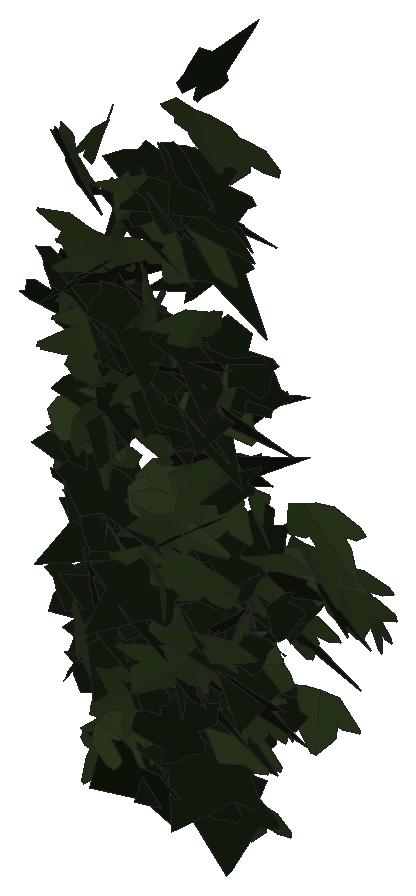
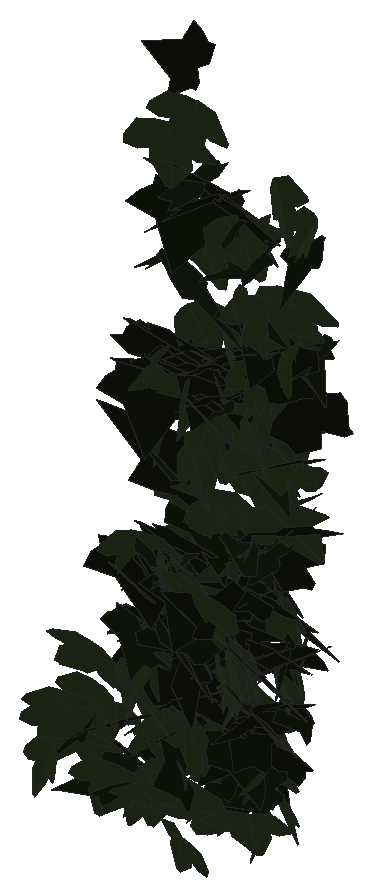
# SketchUp Ruby script. Lengths in millimetres.
U = 1.mm
M = Sketchup.active_model
def pt(a) = Geom::Point3d.new(a.map { |v| v * U })
def face(e, loops, mat)
  f = e.add_face(loops[0].map { |a| pt(a) })
  loops[1..].each { |l| e.add_face(l.map { |a| pt(a) }).erase! }
  f.material = f.back_material = mat if mat
  f
end
# faces: each face lists its corners as indices into pts; further lists are holes
def faces(e, pts, list, mat = nil) = list.each { |f| face(e, (f[0].is_a?(Array) ? f : [f]).map { |l| l.map { |i| pts[i] } }, mat) }
# xy, xz, yz: faces in a plane at the given z, y or x. An outline is a flat list of corners, or four numbers for a rectangle; further outlines are holes
def ring(l) = l.size == 4 ? [[l[0], l[1]], [l[2], l[1]], [l[2], l[3]], [l[0], l[3]]] : l.each_slice(2).to_a
def flat(e, list, mat, &to3) = list.each { |f| face(e, (f[0].is_a?(Array) ? f : [f]).map { |l| ring(l).map { |u, v| to3.(u, v) } }, mat) }
def xy(e, z, list, mat = nil) = flat(e, list, mat) { |x, y| [x, y, z] }
def xz(e, y, list, mat = nil) = flat(e, list, mat) { |x, z| [x, y, z] }
def yz(e, x, list, mat = nil) = flat(e, list, mat) { |y, z| [x, y, z] }
def lines(e, pts, list) = list.each { |a, b| e.add_line(pt(pts[a]), pt(pts[b])) }
# prism: a flat outline (further loops are holes) pulled along v
def prism(e, loops, v, mat = nil)
  f = face(e, loops, mat); d = Geom::Vector3d.new(v.map { |x| x * U })
  f.pushpull(f.normal.samedirection?(d) ? d.length : -d.length)
end
def box(e, o, s, mat = nil) = prism(e, [[o, [o[0] + s[0], o[1], o[2]], [o[0] + s[0], o[1] + s[1], o[2]], [o[0], o[1] + s[1], o[2]]]], [0, 0, s[2]], mat)
def at(x, y, z, deg = 0) = Geom::Transformation.translation(pt([x, y, z])) * Geom::Transformation.rotation(ORIGIN, Z_AXIS, deg.degrees)
def axes(o, x, y, z) = Geom::Transformation.new([*x, 0, *y, 0, *z, 0, *pt(o).to_a, 1])
def part(name) = M.definitions.add(name)
# library, detail: a bought-in or finely detailed component or shape, given as its bounding box
def library(name, o, s) = part(name).tap { |d| box(d.entities, o, s) }
def detail(e, o, s) = box(e.add_group.entities, o, s)
def put(e, d, t, mat = nil) = e.add_instance(d, t).tap { |i| i.material = mat if mat }
def group(e, t, mat = nil) = e.add_group.tap { |g| g.transformation = t; g.material = mat if mat }.entities
root = M.entities
M.materials.add("efeu1").color = [18, 25, 13]
M.materials.add("efeu2").color = [43, 57, 29]
c1 = part("ivyleaf_9")
p = [[39.1,54.8,31.7],[34.5,51.8,30.2],[-5.3,25.2,17.3],[-17.9,28.3,20.9],[-21.6,21.7,17],[-20.2,4.3,5.3],
  [-22.9,-0.3,2.5],[-17.1,-4,-0.6],[-2,-2.1,-1.2],[-0.7,-15.4,-10.1],[16.6,-22.3,-16.7],[21.1,-15.1,-12.5],
  [32.7,-10.7,-11],[46.1,-1.8,-6.6],[30.8,11.2,3.8]]
faces(c1.entities,p,[[0,1,2,3,4,5,6,7,8,9,10,11,12,13,14]],"efeu1")
c2 = part("ivyleaf_10")
p = [[0,12.8,-0.8],[-1.5,51.3,-10.9],[-4.9,51,-11.6],[-13.6,26.5,-7.3],[-13.2,15.9,-4.6],[-21.1,19.3,-7.2],
  [-29.5,16.3,-8.3],[-29.2,8.3,-6.2],[-19.7,-9.8,0.5],[-7.6,-13,4],[1,-12.2,5.8],[-0.4,51.1,-11.1],
  [-1.5,51.1,-10.9],[1,-12.4,5.9],[16.9,-12.4,3.5],[35.1,9.1,-5.1],[35,12.9,-6.1],[20.5,16.4,-4.9],
  [15.8,15,-3.8],[15.3,27.6,-7.1],[12.8,31.3,-7.8]]
faces(c2.entities,p,[[0,1,2,3,4,5,6,7,8,9,10],[11,12,0,13,14,15,16,17,18,19,20]],"efeu2")
put(root,c1,axes([3291.1,941.8,1866.9],[-1.63841,0.20506,-0.06305],[0.10638,-0.03734,-0.88465],[-0.3942,-0.86237,0.02331]))
put(root,c2,axes([3268.6,999.9,1657.1],[1.36446,0.42634,-0.10284],[-0.16436,-0.05598,-0.83411],[-0.81833,0.7221,-0.00394]))
put(root,c2,axes([3261,1111.8,1683.8],[1.21223,-0.44961,0.31681],[0.5749,-0.11914,-0.77639],[0.87479,0.70134,0.07122]))
put(root,c1,axes([3275.5,910.4,1743.9],[0.25103,0.30454,0.864],[0.47233,0.82839,-0.32988],[-1.67833,0.27868,0.03639]))
put(root,c2,axes([3294.5,926.8,1954.7],[-1.01266,-0.47157,0.54848],[-0.75507,-0.37907,-0.71079],[1.1511,-0.66351,0.01627]))
put(root,c2,axes([3274.6,938.9,1874.2],[0.99293,-0.73387,0.02376],[0.02687,-0.01911,-0.90042],[1.39718,0.52191,0.00043]))
put(root,c1,axes([3282.5,919,1826.6],[0.61878,-0.07581,-0.86332],[-1.36691,0.49246,-0.31372],[0.92307,0.78007,0.11416]))
put(root,c2,axes([3278.7,920.6,2128],[-0.11991,-0.82511,0.44369],[0.11724,-0.44737,-0.82322],[1.77912,-0.02613,0.08415]))
put(root,c2,axes([3273.8,968.6,1633.3],[-0.46378,0.81359,-0.01001],[-0.00783,-0.01168,-0.84927],[-1.54853,-0.24361,0.00729]))
put(root,c1,axes([3258,938.2,1814],[0.51924,-0.7897,-0.36067],[0.0588,0.38665,-0.82322],[1.65124,0.23456,0.14273]))
put(root,c1,axes([3245.1,924.3,2070.7],[1.86809,-0.02971,-0.34505],[0.65849,0.12956,0.97308],[0.02888,-1.03233,0.13205]))
put(root,c1,axes([3278.6,892.7,2249.9],[1.08597,-0.13273,-0.74714],[-1.20074,0.43646,-0.55937],[0.80251,0.83266,0.17411]))
put(root,c2,axes([3282,936.3,1650.5],[0.88369,-0.7013,-0.10271],[-0.10379,0.08708,-0.84108],[1.34496,0.4675,0.00258]))
put(root,c2,axes([3280.2,932.8,1781.1],[0.36461,-0.8497,0.28444],[0.16256,-0.27223,-0.87074],[1.69759,0.20857,0.02229]))
put(root,c2,axes([3280.7,935.3,1862.7],[-1.24826,0.57855,-0.19807],[0.06738,-0.25405,-0.85926],[-1.16188,-0.63629,0.16297]))
put(root,c2,axes([3289.5,919,2059.9],[-0.88419,-0.79522,0.11666],[-0.02452,-0.12737,-0.91947],[1.52947,-0.46176,0.0527]))
put(root,c2,axes([3279.4,959.6,1655.2],[-0.30491,0.82154,-0.12098],[0.02656,-0.12053,-0.83696],[-1.58019,-0.16055,0.00928]))
put(root,c1,axes([3269.8,945,1754.5],[0.52384,-0.21759,-0.79415],[-0.233,0.81722,-0.26634],[1.5497,0.19642,0.2284]))
put(root,c1,axes([3284.4,1083.7,1737.7],[0.29329,0.23543,0.82329],[0.48535,0.78594,-0.27248],[-1.55574,0.28958,0.0702]))
put(root,c1,axes([3285.8,933.1,1942.7],[-0.99855,-0.73699,0.09525],[-0.04457,-0.10014,-0.90384],[1.4136,-0.52376,0.03878]))
put(root,c1,axes([3301.4,885,2144.4],[-0.25789,0.93298,0.12548],[-0.0107,0.12597,-0.94269],[-1.79161,-0.13505,-0.01243]))
put(root,c2,axes([3281.1,968.4,1689.2],[-0.26334,0.83743,0.04284],[0.00062,0.04347,-0.84875],[-1.59589,-0.13817,-0.0074]))
put(root,c2,axes([3300.7,896.4,2178.8],[-1.69504,0.05393,0.30576],[-0.58094,0.01773,-0.89226],[-0.10803,-0.94148,0.00072]))
put(root,c1,axes([3263.5,970.7,1680.9],[1.19495,-0.56293,-0.03573],[0.04025,0.07691,-0.84025],[1.07278,0.62416,0.07132]))
put(root,c2,axes([3291,915.5,2065.8],[-1.09684,-0.75007,0.02522],[0.13556,-0.08632,-0.93961],[1.4219,-0.57037,0.10903]))
put(root,c1,axes([3265.3,909,2130.1],[0.61208,-0.89231,0.10139],[0.09667,-0.08945,-0.94834],[1.70644,0.32513,0.01736]))
put(root,c2,axes([3285.1,888.8,2265.1],[-0.9256,0.81522,0.00802],[0.01029,0.01257,-0.9492],[-1.55156,-0.48624,-0.01108]))
put(root,c1,axes([3287.3,957.2,1750.5],[-0.68087,-0.74381,0.21767],[-0.18868,-0.19385,-0.82535],[1.46287,-0.3712,-0.00515]))
put(root,c1,axes([3318,956.8,1807],[-0.96334,0.64874,0.28351],[-0.41672,0.18798,-0.82107],[-1.28137,-0.54886,0.05388]))
put(root,c1,axes([3276,922,1946.9],[0.70388,-0.75674,-0.35005],[-0.31631,0.30835,-0.84218],[1.555,0.40527,-0.01286]))
put(root,c2,axes([3273.2,913.3,1782.4],[0.19932,-0.36689,0.82699],[1.12123,-0.60416,-0.34264],[1.30678,0.57434,0.16785]))
put(root,c1,axes([3270.6,959.7,1721.2],[-0.41494,-0.23195,-0.79436],[1.39421,0.32799,-0.29684],[0.73256,-0.75562,0.115]))
put(root,c2,axes([3281.8,905.4,1999.4],[0.82313,0.71572,0.44173],[0.40911,0.38615,-0.83613],[-1.54755,0.48277,0.01391]))
put(root,c2,axes([3302.1,883.4,2001.3],[0.17706,0.56348,0.72436],[-0.56728,0.70716,-0.51182],[-1.65192,-0.18244,0.2534]))
put(root,c1,axes([3313.5,966,1710.4],[-0.17603,0.83843,-0.1339],[0.00078,-0.13465,-0.8434],[-1.61592,-0.0914,0.01418]))
put(root,c1,axes([3323.1,959.9,1768],[-1.11865,0.61618,0.06786],[-0.11089,0.03819,-0.85141],[-1.17458,-0.59044,0.01575]))
put(root,c2,axes([3306.1,915.7,2093.8],[-0.93168,-0.7833,0.20194],[0.02648,-0.24416,-0.91333],[1.53929,-0.4699,0.13794]))
put(root,c2,axes([3308,929.5,2015.3],[-1.50879,-0.45023,-0.02683],[0.03169,0.025,-0.91159],[0.8578,-0.79282,-0.01351]))
put(root,c1,axes([3312.4,948.2,1814.8],[-1.60594,-0.19726,-0.18221],[0.36375,-0.0191,-0.86443],[0.35901,-0.86305,0.06078]))
put(root,c2,axes([3312.7,920.1,2106],[-1.39002,-0.58311,0.05549],[-0.08609,-0.03227,-0.93458],[1.11146,-0.73175,-0.003]))
put(root,c2,axes([3309,909.9,2154.5],[-0.96161,-0.80101,-0.05026],[0.12091,0.01929,-0.94606],[1.5227,-0.50739,0.04338]))
put(root,c1,axes([3288.1,933.6,1881.1],[0.5229,-0.80355,-0.27842],[-0.04352,0.2855,-0.84656],[1.61793,0.26738,0.06721]))
put(root,c2,axes([3308.5,956.7,1805.5],[0.54209,-0.82276,-0.06216],[0.00712,0.06705,-0.8703],[1.57032,0.28372,0.02541]))
put(root,c1,axes([3301.8,929.3,2007.2],[-0.68627,-0.83056,0.17307],[0.01472,-0.19126,-0.90176],[1.61461,-0.35128,0.08178]))
put(root,c1,axes([3270.7,917.7,1904.5],[1.12013,-0.42318,0.60133],[0.99188,-0.30329,-0.72352],[0.98723,0.78486,0.04464]))
put(root,c1,axes([3285.9,937.9,1915.6],[0.86805,-0.77566,-0.00192],[0.03362,0.01262,-0.89956],[1.47586,0.45593,0.02162]))
put(root,c2,axes([3317.8,912.2,1725.1],[1.03158,-0.50406,-0.50402],[-0.49408,0.45011,-0.72932],[1.26347,0.58756,0.12631]))
put(root,c1,axes([3271.5,922.9,2119.9],[1.27182,-0.28484,0.59393],[1.03542,-0.23831,-0.72641],[0.70675,0.8617,-0.00457]))
put(root,c1,axes([3299.2,926.7,1810.4],[-0.88287,-0.57428,-0.502],[0.6088,0.38692,-0.73822],[1.31786,-0.56347,0.00472]))
put(root,c1,axes([3297.5,966,1728.6],[1.66358,-0.12322,-0.31616],[-0.59212,0.05772,-0.88264],[0.2578,0.92772,0.01292]))
put(root,c2,axes([3300.2,1106.5,1726.4],[0.63414,0.76213,0.286],[0.20342,0.2654,-0.83175],[-1.53584,0.34983,0.00792]))
put(root,c2,axes([3315.1,892.7,2294.3],[0.05351,-0.9489,-0.20865],[0.02754,0.20912,-0.9491],[1.84888,0.02435,0.02018]))
put(root,c2,axes([3331.9,919.7,1689.6],[0.9452,-0.30401,-0.70783],[-1.09882,0.41067,-0.58147],[0.97065,0.76094,0.03102]))
put(root,c2,axes([3310.7,964.3,1772.3],[-0.82074,0.74065,0.05517],[-0.03569,0.05292,-0.85699],[-1.41307,-0.43153,-0.0104]))
put(root,c1,axes([3332.8,906.9,1995.8],[0.00541,0.77291,0.49877],[-0.51778,0.47716,-0.73788],[-1.67237,-0.14523,0.23006]))
put(root,c1,axes([3332.7,932,1912.6],[-0.90542,0.73736,-0.16871],[0.03254,-0.18877,-0.87325],[-1.43924,-0.46814,0.08639]))
put(root,c2,axes([3318.3,912.3,2169.1],[-1.57743,-0.45028,-0.04002],[0.04335,0.04187,-0.94289],[0.85926,-0.82874,-0.0259]))
put(root,c1,axes([3309.5,956.4,1801.4],[-0.55279,-0.77516,0.27355],[-0.00975,-0.28842,-0.82272],[1.56443,-0.2757,0.09153]))
put(root,c2,axes([3298.3,1082,1736.7],[-0.65088,0.40064,-0.69592],[0.79107,-0.55886,-0.526],[-1.3076,-0.53752,0.02819]))
put(root,c2,axes([3321.9,922,2044.9],[-0.22531,-0.92552,-0.06851],[0.0021,0.06893,-0.93303],[1.76626,-0.11814,-0.00763]))
put(root,c1,axes([3315.2,917.8,2123.7],[-0.7669,-0.85604,0.03989],[-0.02356,-0.03825,-0.94612],[1.63081,-0.40311,0.00509]))
put(root,c2,axes([3322.6,956.4,1799.8],[0.20143,-0.86488,-0.05368],[0.00093,0.05414,-0.8713],[1.6492,0.1056,0.00705]))
put(root,c1,axes([3319.6,897.8,2149.4],[0.80267,0.82441,0.1255],[0.13236,0.10537,-0.92592],[-1.58156,0.42722,-0.0138]))
put(root,c2,axes([3308.3,902.2,1987.4],[1.05478,-0.62262,0.39865],[0.68387,-0.20857,-0.8253],[1.22968,0.65006,0.11703]))
put(root,c1,axes([3303.2,892.5,1946.4],[0.69392,-0.78084,-0.35188],[0.04665,0.39179,-0.84402],[1.62936,0.32133,0.17402]))
put(root,c2,axes([3321.1,1097.7,1717.5],[-0.06378,0.79231,-0.3833],[-0.03994,-0.38419,-0.79232],[-1.67465,-0.02102,0.03349]))
put(root,c1,axes([3321.8,937.3,1662.9],[1.47789,-0.04593,-0.47015],[-0.89144,0.04255,-0.77778],[0.11669,0.90677,0.01268]))
put(root,c2,axes([3330.6,963.1,1790.5],[0.2883,-0.84444,-0.06332],[-0.00089,0.06424,-0.85785],[1.61165,0.15109,0.01085]))
put(root,c1,axes([3341.5,948,1710.3],[-1.55135,-0.24427,-0.00506],[0.00894,0.00197,-0.85094],[0.46491,-0.81514,-0.00054]))
put(root,c2,axes([3327.3,964.6,1716.1],[-0.83099,-0.6273,-0.38671],[0.37417,0.33404,-0.76384],[1.35167,-0.47812,-0.0263]))
put(root,c1,axes([3319.8,898,2033.5],[1.01509,-0.38539,-0.68611],[-0.71566,0.60329,-0.63118],[1.31566,0.62551,0.18603]))
put(root,c2,axes([3329.6,1090.7,1832.1],[-0.5716,0.79558,0.16934],[-0.12887,0.15543,-0.85035],[-1.5427,-0.30776,0.00829]))
put(root,c2,axes([3326.1,937.8,1906.9],[0.03479,0.8674,-0.26461],[0.00982,-0.26476,-0.86753],[-1.72592,0.01598,-0.01027]))
put(root,c1,axes([3325.3,961,1673.4],[1.17675,-0.36653,-0.46491],[-0.72696,0.26662,-0.71819],[0.86084,0.72619,0.02903]))
put(root,c2,axes([3331.2,929.8,1674.3],[-0.03022,-0.12607,-0.94432],[0.43653,0.91617,-0.12617],[1.75985,-0.22942,0.01508]))
put(root,c2,axes([3324.7,896.5,1698],[0.22969,0.64943,0.6144],[0.23018,0.60241,-0.66052],[-1.68583,0.17073,-0.00647]))
put(root,c2,axes([3323.4,953.8,1810.7],[1.30474,-0.47728,0.27133],[0.53186,-0.07027,-0.82967],[0.89939,0.73393,0.09701]))
put(root,c2,axes([3328.4,925.1,1985.2],[-0.00025,-1.00563,-0.30699],[0.08299,-0.30673,1.00477],[-1.9994,-0.0126,0.04174]))
put(root,c1,axes([3357.7,889.6,1677.5],[0.75096,0.07969,-0.90298],[-1.69747,-0.14185,-0.40226],[-0.30828,0.97517,0.01528]))
put(root,c1,axes([3343.5,1090.4,1820.9],[-1.268,0.29278,-0.48853],[0.83344,-0.21737,-0.72749],[-0.69306,-0.79705,0.01895]))
put(root,c1,axes([3347.2,952.1,1826.4],[-1.436,-0.4577,-0.00553],[0.01024,0.00179,-0.88249],[0.87109,-0.75454,0.00126]))
put(root,c2,axes([3344.7,934.9,1746.7],[-1.29077,-0.57029,-0.05161],[0.06775,0.03786,-0.88609],[1.08769,-0.67912,-0.00605]))
put(root,c2,axes([3335.4,955.6,1770.7],[-0.81675,0.70692,-0.22816],[0.18408,-0.20808,-0.82663],[-1.40172,-0.43924,0.02439]))
put(root,c1,axes([3323.9,904.9,2094.8],[0.92761,-0.71309,-0.3513],[-0.28245,0.3232,-0.86196],[1.4863,0.50647,0.05544]))
put(root,c1,axes([3320.5,926.8,1872.5],[1.70449,-0.12999,-0.0139],[-0.02625,0.00174,-0.90498],[0.24742,0.8957,-0.00026]))
put(root,c2,axes([3313.7,1005.5,1653.6],[0.47184,-0.07685,0.80375],[1.40922,0.3569,-0.19427],[-0.61275,0.76164,0.17213]))
put(root,c2,axes([3349.5,1111.7,1727.8],[-1.60537,0.0756,-0.06583],[0.12402,-0.01043,-0.84688],[-0.14498,-0.84601,0.00456]))
put(root,c2,axes([3357.5,929.6,1865.7],[-0.83895,-0.72991,0.3487],[-0.14927,-0.35668,-0.84575],[1.53229,-0.43438,0.10853]))
put(root,c2,axes([3362.3,908.8,2242],[-0.91767,-0.75284,0.31794],[-0.33781,-0.26387,-0.89399],[1.51822,-0.51376,-0.00674]))
put(root,c1,axes([3363.2,899.5,1854.1],[-1.61506,0.08778,-0.20637],[0.37512,-0.09341,-0.8502],[-0.20362,-0.86832,0.0706]))
put(root,c2,axes([3353.8,922,2031.2],[-0.87034,-0.8071,0.09596],[0.13713,-0.14992,-0.91764],[1.54079,-0.44256,0.13587]))
put(root,c2,axes([3348.6,877.7,2227.6],[-0.0317,-0.10873,-1.00511],[0.34096,0.98902,-0.10996],[1.89363,-0.1799,0.00297]))
put(root,c1,axes([3329.8,900.2,2224],[1.17699,-0.72069,-0.18351],[-0.18376,0.15884,-0.94919],[1.4034,0.62522,0.02962]))
put(root,c1,axes([3335.5,947.3,1834.5],[-0.04791,-0.03366,0.87772],[1.41859,0.46373,0.03916],[-0.88442,0.74564,0.01527]))
put(root,c1,axes([3339,899.5,1821.2],[1.47869,-0.3726,-0.43778],[-0.61795,0.32297,-0.85112],[0.90289,0.83126,0.13445]))
put(root,c2,axes([3358.3,912.9,2126.3],[0.16979,-0.94739,-0.00917],[-0.00675,0.00888,-0.95157],[1.80314,0.08924,-0.0027]))
put(root,c2,axes([3357.2,942.7,1723.6],[0.86027,-0.75716,-0.05301],[-0.07894,0.03696,-0.88166],[1.44239,0.45361,-0.01664]))
put(root,c1,axes([3345.8,907.4,2116.3],[-0.32995,-0.91347,0.07339],[-0.01505,-0.0732,-0.92976],[1.74405,-0.17345,0.00586]))
put(root,c2,axes([3341.8,919.8,1668],[-1.40074,-0.15467,-0.52759],[1.00012,0.06129,-0.75104],[0.30765,-0.90348,0.03937]))
put(root,c2,axes([3372.9,886.3,2142.8],[-0.02918,-0.01827,-1.01117],[-0.46256,0.98171,-0.01405],[1.86836,0.24276,-0.01927]))
put(root,c2,axes([3356.9,896.6,2060.8],[-0.41427,-0.75169,-0.50229],[0.40893,0.45882,-0.77975],[1.67131,-0.29859,0.06629]))
put(root,c1,axes([3356.3,921.8,2064.2],[-0.76356,-0.8429,0.05079],[0.03041,-0.0638,-0.93258],[1.60684,-0.39934,0.04179]))
put(root,c1,axes([3341.5,934.4,1735.3],[0.61412,-0.82099,-0.07439],[-0.00392,0.07908,-0.88172],[1.56891,0.32156,0.02692]))
put(root,c2,axes([3366.6,912.4,2013.5],[-1.45106,-0.48851,-0.03012],[0.04291,0.02065,-0.90549],[0.93052,-0.76275,-0.00522]))
put(root,c2,axes([3358.3,952.1,1834.8],[-1.25872,0.53417,-0.20947],[0.3057,-0.1345,-0.85014],[-1.04834,-0.68059,0.00361]))
put(root,c1,axes([3389.7,918.9,1847.5],[0.33893,-0.1101,0.87837],[-1.37289,0.5013,0.20908],[-0.97659,-0.74294,0.01091]))
put(root,c1,axes([3390.2,966.8,1763.8],[0.17241,0.26322,-0.81336],[-1.19944,-0.53209,-0.24239],[-1.09936,0.62181,0.1369]))
put(root,c1,axes([3361,964.5,1744.4],[-0.62914,-0.7898,-0.03349],[0.0133,0.03338,-0.85616],[1.50444,-0.33058,-0.00643]))
put(root,c1,axes([3341.5,1107.5,1726.1],[1.16585,-0.58574,0.00179],[0.12805,0.06779,-0.84215],[1.10741,0.60882,0.09549]))
put(root,c2,axes([3366.6,957.6,1742.7],[1.41272,-0.41948,-0.09639],[-0.14079,0.06497,-0.85238],[0.80697,0.74569,0.02003]))
put(root,c1,axes([3379.3,901.4,2260.8],[-1.73228,0.1357,-0.27704],[0.53021,-0.00914,-0.91974],[-0.25218,-0.95138,-0.03068]))
put(root,c1,axes([3362.4,1109.2,1777.8],[-0.52348,-0.82833,0.16934],[-0.03346,-0.17243,-0.87202],[1.60874,-0.27313,0.03697]))
put(root,c2,axes([3375.9,929.5,1824.7],[-0.60649,-0.76691,0.29919],[-0.08789,-0.30366,-0.82757],[1.56425,-0.31441,0.0695]))
put(root,c2,axes([3387.3,910.2,1782.3],[-1.10307,-0.55475,0.46155],[-0.64593,-0.31289,-0.80226],[1.21207,-0.6716,-0.00749]))
put(root,c1,axes([3368.9,921.6,1652.5],[-0.43729,-0.33,0.7627],[-0.39107,-0.74418,-0.38389],[1.53249,-0.28407,0.11967]))
put(root,c1,axes([3396.1,915.7,2031.1],[-1.34188,0.5943,0.03616],[-0.04697,0.02683,-0.92211],[-1.13219,-0.70548,-0.0046]))
put(root,c1,axes([3336.3,956.6,1806.8],[0.72919,-0.14045,0.77192],[1.38142,-0.26273,-0.40807],[0.56698,0.82075,0.00147]))
put(root,c1,axes([3383.4,962.9,1782.1],[0.8626,0.00637,-0.73237],[-1.38965,0.0711,-0.45126],[0.10871,0.85833,0.04282]))
put(root,c1,axes([3366.1,913.7,2094.4],[-0.65154,-0.88233,0.07973],[0.02593,-0.09071,-0.94532],[1.68588,-0.33959,0.04535]))
put(root,c2,axes([3382,963.9,1700.8],[-1.59145,0.14038,0.1333],[-0.25963,-0.00794,-0.84737],[-0.26141,-0.84672,0.03005]))
put(root,c2,axes([3351.4,971.2,1861.6],[1.68399,-0.08092,0.52092],[0.99216,-0.01699,-0.88812],[0.14914,1.02663,0.02636]))
put(root,c1,axes([3362.5,922.2,2044.6],[-1.05735,-0.32246,-0.65463],[1.15831,0.2492,-0.63927],[0.76629,-0.82164,0.06303]))
put(root,c2,axes([3359.9,920.9,1937.8],[1.0533,0.69538,0.34378],[0.44722,0.25218,-0.88838],[-1.40698,0.60074,-0.02501]))
put(root,c1,axes([3373,943.1,1849.9],[1.04287,0.68663,0.03417],[0.01142,0.03892,-0.87826],[-1.30837,0.54764,0.01957]))
put(root,c2,axes([3382.3,885.9,1873.8],[0.78526,-0.49873,-0.61269],[-0.16628,0.65818,-0.59458],[1.49433,0.33532,0.25581]))
put(root,c1,axes([3399.6,933.1,1860.8],[-0.69071,0.81419,0.14316],[-0.14657,0.12237,-0.89119],[-1.5665,-0.37045,0.02026]))
put(root,c2,axes([3379.2,952.7,1790.5],[0.99156,-0.68456,-0.04577],[0.02053,0.06564,-0.85891],[1.3056,0.51887,0.04827]))
put(root,c2,axes([3381.1,903.9,1922.7],[-0.99949,-0.74176,-0.23016],[0.2995,0.17044,-0.90838],[1.44746,-0.54746,0.02903]))
put(root,c2,axes([3375.3,932.6,1952.3],[1.50695,0.44741,-0.06621],[-0.09555,-0.04571,-0.90934],[-0.85546,0.79325,-0.01505]))
put(root,c2,axes([3377.9,1103.6,1791],[1.53022,0.37325,-0.09895],[-0.20374,-0.00414,-0.88548],[-0.70609,0.81008,0.04107]))
put(root,c1,axes([3370,951.1,1842.3],[-0.21699,-0.85111,0.18479],[0.03028,-0.18837,-0.85779],[1.65729,-0.10799,0.03987]))
put(root,c1,axes([3354,952.6,1797.3],[1.31567,-0.52178,0.14899],[0.31042,-0.03034,-0.86303],[0.98498,0.70652,0.07297]))
put(root,c1,axes([3354.2,959,1818.9],[1.50536,-0.33008,0.15479],[0.37799,0.08003,-0.84421],[0.58186,0.80198,0.14795]))
put(root,c2,axes([3375.7,923.9,1799.1],[-1.31287,0.39589,-0.33862],[0.42644,-0.28179,-0.7859],[-0.8951,-0.71492,0.12226]))
put(root,c1,axes([3411.7,1009,1683.8],[-0.42043,0.53378,0.63302],[-0.868,0.46839,-0.55412],[-1.31532,-0.47972,0.16333]))
put(root,c2,axes([3384.2,938.6,1790.2],[1.00437,-0.68683,-0.0084],[-0.01498,0.00454,-0.86615],[1.30719,0.52777,-0.00347]))
put(root,c1,axes([3402.6,952.2,1801.9],[-0.56964,0.79821,0.13763],[-0.04031,0.13896,-0.852],[-1.54104,-0.29869,-0.02859]))
put(root,c2,axes([3356,906.6,1923.5],[-0.76616,-0.10954,-0.83439],[1.59863,-0.10885,-0.39097],[-0.09792,-0.92,0.1456]))
put(root,c1,axes([3415.3,895.9,1731.2],[-1.10588,0.65738,0.34874],[-0.46049,0.25152,-0.87726],[-1.33932,-0.62927,0.01367]))
put(root,c2,axes([3390.5,903.2,2076.1],[0.58372,-0.88746,-0.15027],[-0.09083,0.14249,-0.93896],[1.71064,0.31039,0.00142]))
put(root,c2,axes([3391.8,930.9,1989.2],[-0.32622,-0.89668,-0.00621],[0.02403,0.00391,-0.91284],[1.70643,-0.17147,0.01167]))
put(root,c2,axes([3384.3,1099.5,1802.8],[-1.41399,0.38886,-0.17377],[0.23764,-0.13518,-0.83637],[-0.77498,-0.75093,0.06058]))
put(root,c1,axes([3384.3,949.4,1756.1],[-0.50053,-0.79086,0.24415],[-0.16873,-0.22778,-0.83336],[1.56619,-0.27729,-0.01176]))
put(root,c1,axes([3400.6,906.3,1917.5],[0.03218,0.94048,-0.03148],[-0.00058,-0.03148,-0.94063],[-1.79092,0.01691,-0.00026]))
put(root,c1,axes([3372.7,895.3,2248.9],[1.31503,-0.54814,-0.36589],[-0.50797,0.25197,-0.88149],[1.14683,0.74014,0.02911]))
put(root,c1,axes([3365.2,911.3,2056.1],[0.93634,-0.77447,0.10572],[0.14302,-0.07748,-0.91727],[1.48076,0.49721,0.02174]))
put(root,c1,axes([3425,930.2,1654.6],[-0.57186,0.08024,0.86489],[-1.63293,0.11523,-0.30876],[-0.25767,-0.90832,0.03723]))
put(root,c2,axes([3416.4,904.7,1880.5],[-1.37538,-0.23715,0.5618],[-0.96073,-0.25608,-0.75744],[0.65111,-0.8788,0.06911]))
put(root,c2,axes([3398.4,963.2,1768.2],[-1.34717,-0.48872,-0.01651],[0.04464,-0.00492,-0.86],[0.9296,-0.70802,0.01737]))
put(root,c1,axes([3391.6,949.2,1853.4],[-0.91547,-0.73637,-0.10209],[0.18697,0.05757,-0.87811],[1.40246,-0.48835,0.05042]))
put(root,c1,axes([3394.3,897.1,2080.1],[1.12748,0.75239,-0.08961],[-0.08789,-0.07768,-0.95755],[-1.43939,0.59409,-0.01172]))
put(root,c2,axes([3397.7,947.8,1866.6],[1.30583,-0.55,-0.06522],[-0.11378,0.02969,-0.87924],[1.04793,0.68858,-0.01419]))
put(root,c1,axes([3424.2,915.8,2184.6],[-1.10019,0.85894,-0.08509],[0.09404,-0.06931,-1.03534],[-1.64004,-0.58018,-0.00229]))
put(root,c2,axes([3403.6,945,1850.3],[-1.63749,0.19813,-0.04154],[0.05496,-0.0594,-0.88141],[-0.38135,-0.85934,0.05135]))
put(root,c2,axes([3402.4,925,2054.9],[0.05996,-0.75243,-0.5322],[0.23856,0.53106,-0.7434],[1.73773,-0.04694,0.12042]))
put(root,c1,axes([3394.1,1099.7,1775.5],[1.13667,-0.43254,-0.50281],[-0.76908,0.29923,-0.73741],[1.00097,0.72109,0.00439]))
put(root,c1,axes([3386.2,963.8,1702.5],[0.37636,-0.83605,0.00887],[0.03445,-0.00483,-0.85896],[1.59088,0.19789,0.0165]))
put(root,c2,axes([3410,906.8,2129],[-0.5302,-0.86412,0.23379],[-0.00492,-0.24407,-0.90521],[1.70372,-0.26962,0.07014]))
put(root,c2,axes([3390.4,1095.5,1844.8],[-1.30508,0.09576,-0.51688],[0.79734,-0.41361,-0.63243],[-0.6043,-0.75254,0.28182]))
put(root,c1,axes([3379.8,929.4,1754.8],[0.93737,-0.69361,0.12402],[0.21377,-0.07209,-0.84926],[1.32387,0.50276,0.04932]))
put(root,c2,axes([3379.8,951.9,1727.7],[-0.47366,-0.22454,0.81622],[1.21485,0.50903,0.33467],[-1.05824,0.68486,0.01886]))
put(root,c2,axes([3408.8,1141.9,1744.3],[-1.05329,0.68034,0.10155],[-0.1713,0.0576,-0.87638],[-1.29792,-0.55972,0.03325]))
put(root,c2,axes([3401.7,896.6,1960.7],[0.41059,-0.63239,-0.65166],[0.4682,0.68545,-0.58374],[1.66358,-0.03683,0.32512]))
put(root,c2,axes([3402.7,1110.9,1786.4],[-1.54974,-0.09115,-0.26165],[0.49141,0.04501,-0.81922],[0.19129,-0.8541,-0.01525]))
put(root,c1,axes([3431,932,1890.8],[-1.68409,0.07931,0.06994],[-0.13796,-0.02589,-0.88784],[-0.14652,-0.88725,0.03216]))
put(root,c1,axes([3393.5,938.6,1721.8],[0.5829,-0.50665,-0.6268],[-0.19578,0.64048,-0.56797],[1.52136,0.27654,0.16706]))
put(root,c2,axes([3412.2,1108,1768.8],[-1.60731,-0.1361,-0.05055],[0.08983,0.02474,-0.85526],[0.2613,-0.84568,-0.01689]))
put(root,c2,axes([3414,947.6,1869.8],[0.10377,-0.88445,-0.07136],[-0.02845,0.07057,-0.88607],[1.68852,0.05554,-0.01054]))
put(root,c2,axes([3413.6,896.4,2212],[1.75096,-0.16495,-0.2351],[-0.38014,0.19943,-0.92154],[0.39275,0.9284,0.15618]))
put(root,c2,axes([3415.6,925,1943.5],[1.61702,-0.22571,-0.25975],[-0.45139,0.11724,-0.87766],[0.47452,0.88068,0.05027]))
put(root,c2,axes([3412.4,917,1806.6],[-1.68824,-0.12652,-0.11291],[0.21363,0.01265,-0.89602],[0.2419,-0.89412,0.0033]))
put(root,c2,axes([3422.6,961.4,1632.6],[-1.57959,0.16103,0.1785],[-0.33051,0.04207,-0.8454],[-0.31638,-0.8479,-0.00804]))
put(root,c1,axes([3394.2,894.4,2261],[0.58386,-0.66818,-0.61278],[-0.03341,0.64241,-0.70928],[1.72516,0.23858,0.19365]))
put(root,c1,axes([3443.5,899.4,2277.1],[-1.81478,0.13908,0.1557],[-0.32018,-0.08078,-0.95813],[-0.2353,-0.96279,0.10288]))
put(root,c2,axes([3404.6,925.3,1702.4],[1.78317,0.16638,0.14697],[0.27017,0.04108,-0.95147],[-0.32483,0.9475,0.01544]))
put(root,c1,axes([3396,915.7,2040.3],[0.17834,-0.92083,-0.09485],[0.29727,0.10969,-0.91064],[1.73653,0.07579,0.16563]))
put(root,c1,axes([3435.4,940.3,1814.8],[-1.63258,0.1344,-0.06234],[0.09672,-0.07711,-0.8656],[-0.26486,-0.85661,0.06814]))
put(root,c2,axes([3425.1,918.3,1982.5],[-0.66542,-0.80997,0.20365],[-0.11045,-0.19668,-0.88188],[1.58567,-0.3536,0.02403]))
put(root,c1,axes([3397.7,944.8,1872.9],[0.84056,-0.72964,-0.25832],[-0.09674,0.26943,-0.84793],[1.46994,0.43497,0.09191]))
put(root,c1,axes([3406.8,915.1,2099.9],[-0.27317,-0.88987,0.27389],[0.04742,-0.2807,-0.89892],[1.77136,-0.12972,0.0663]))
put(root,c1,axes([3420.2,896.7,2248.6],[1.49064,0.42115,-0.40357],[-0.92544,0.09824,-0.84118],[-0.61315,0.87559,0.28849]))
put(root,c2,axes([3429.5,960.5,1732.9],[-1.44622,0.37137,0.1778],[-0.46658,-0.10825,-0.82167],[-0.62958,-0.77287,0.20052]))
put(root,c1,axes([3426.7,910.9,1694.5],[-1.23752,-0.62372,0.01385],[-0.01055,-0.01423,-0.90099],[1.18731,-0.65022,0.00643]))
put(root,c1,axes([3422.4,919.1,2073.6],[-1.37937,-0.51666,-0.29892],[0.49599,0.14912,-0.88962],[1.02203,-0.76967,0.0283]))
put(root,c1,axes([3400.1,910.6,2281.2],[0.75396,-0.86843,0.04033],[0.07346,-0.0267,-0.95422],[1.65294,0.39731,0.02401]))
put(root,c1,axes([3440.6,938.5,1878.8],[-1.09251,0.52944,-0.42353],[0.25962,-0.45341,-0.75168],[-1.26398,-0.55074,0.21168]))
put(root,c1,axes([3437.1,939,1835.6],[-0.56236,0.60973,-0.55694],[0.24605,-0.55007,-0.6708],[-1.55229,-0.30808,0.09544]))
put(root,c1,axes([3417.3,933.2,1652],[-0.97566,-0.63793,-0.33703],[0.45062,0.2418,-0.81781],[1.29709,-0.56385,0.0306]))
put(root,c1,axes([3446.8,923.3,1976],[-1.21829,0.64987,-0.10604],[0.01321,-0.14122,-0.90738],[-1.25311,-0.63329,0.09353]))
put(root,c1,axes([3439.7,931,1865.7],[-0.80417,0.57344,-0.53397],[0.25931,-0.54364,-0.69165],[-1.46854,-0.41001,0.17027]))
put(root,c1,axes([3454,912.8,2067.5],[0.16546,0.0547,0.94184],[-1.62413,0.40785,0.05508],[-0.76558,-0.85339,0.08669]))
put(root,c1,axes([3394.2,925,1969.5],[1.42225,0.66545,-0.25331],[0.3209,0.19138,1.00019],[1.3166,-0.7655,0.02986]))
put(root,c1,axes([3433.7,961.2,1791.3],[0.3444,0.72038,0.44001],[0.0572,0.44422,-0.73964],[-1.60553,0.17036,0.06804]))
put(root,c2,axes([3425.5,940.4,1868.1],[-0.87621,0.75729,-0.00295],[-0.00194,-0.00407,-0.88625],[-1.44129,-0.46038,0.00299]))
put(root,c2,axes([3431.1,887.9,2341.4],[-1.73346,0.30113,-0.00657],[-0.00295,-0.02561,-0.95898],[-0.57323,-0.91048,0.0248]))
put(root,c2,axes([3458.7,945.1,1790.5],[-0.79282,0.26358,0.71128],[-1.44205,-0.18299,-0.37595],[0.06831,-0.80372,0.31886]))
put(root,c2,axes([3415.9,912.6,2050.2],[0.62512,0.66171,0.55842],[0.35413,0.52935,-0.73671],[-1.60937,0.3735,0.05479]))
put(root,c1,axes([3449,922.3,2104.8],[-1.76803,0.01646,-0.0363],[0.06898,-0.00378,-0.92912],[-0.03159,-0.92968,0.00313]))
put(root,c2,axes([3422,958.6,1694.5],[-0.0625,-0.68861,-0.52327],[0.62903,0.47391,-0.6444],[1.52109,-0.22428,0.24498]))
put(root,c1,axes([3393.4,910.4,2051.5],[1.05999,-0.43869,0.65103],[0.99705,-0.38681,-0.70882],[1.11276,0.76448,0.01495]))
put(root,c1,axes([3440.9,951.6,1869.5],[0.9823,0.58276,-0.41597],[-0.54444,-0.30222,-0.77836],[-1.24917,0.58998,0.01215]))
put(root,c2,axes([3446.6,906.3,2318.3],[-1.79282,0.03054,0.18132],[-0.34535,-0.00156,-0.94247],[-0.05651,-0.95929,0.00731]))
put(root,c2,axes([3437.3,943.4,1839.1],[-0.214,0.3847,-0.77795],[-0.15512,-0.78567,-0.37674],[-1.64444,0.02405,0.13678]))
put(root,c1,axes([3444.8,931.9,2048.6],[0.60417,0.86349,0.0264],[0.01637,0.02496,-0.92],[-1.64408,0.31757,0.00054]))
put(root,c1,axes([3422,908.9,2204.3],[0.53114,-0.90035,-0.1745],[-0.00365,0.18183,-0.94122],[1.74542,0.27436,0.05113]))
put(root,c2,axes([3452.6,956.7,1744.5],[-0.85712,0.52077,0.53425],[-0.64634,0.41255,-0.68842],[-1.2643,-0.56396,-0.01025]))
put(root,c1,axes([3463.6,959,1847.4],[-1.46451,0.40234,-0.05586],[0.09682,-0.02325,-0.86833],[-0.76699,-0.77117,-0.00296]))
put(root,c1,axes([3422.1,925.8,1769.4],[1.7055,-0.10876,-0.00098],[-0.00171,0.00072,-0.9027],[0.207,0.89612,0.00061]))
put(root,c1,axes([3435.6,876.9,2385.9],[0.05118,-0.13384,0.95916],[1.18118,0.73899,0.08572],[-1.41495,0.61205,0.10625]))
put(root,c2,axes([3436.9,1035.9,1705.3],[1.59137,-0.15349,0.13647],[0.25925,-0.01375,-0.85006],[0.29256,0.84711,0.01093]))
put(root,c1,axes([3442,941.3,1792],[-0.67975,-0.82388,0.04236],[0.00051,-0.04628,-0.89777],[1.57008,-0.35668,0.01863]))
put(root,c2,axes([3446.1,950.8,1882.1],[-1.18167,-0.58095,-0.19488],[0.33142,0.09871,-0.84907],[1.11814,-0.64322,0.04572]))
put(root,c2,axes([3442,912,2071.7],[0.00571,-0.3785,-0.84862],[0.58973,0.80046,-0.35592],[1.66724,-0.28184,0.1288]))
